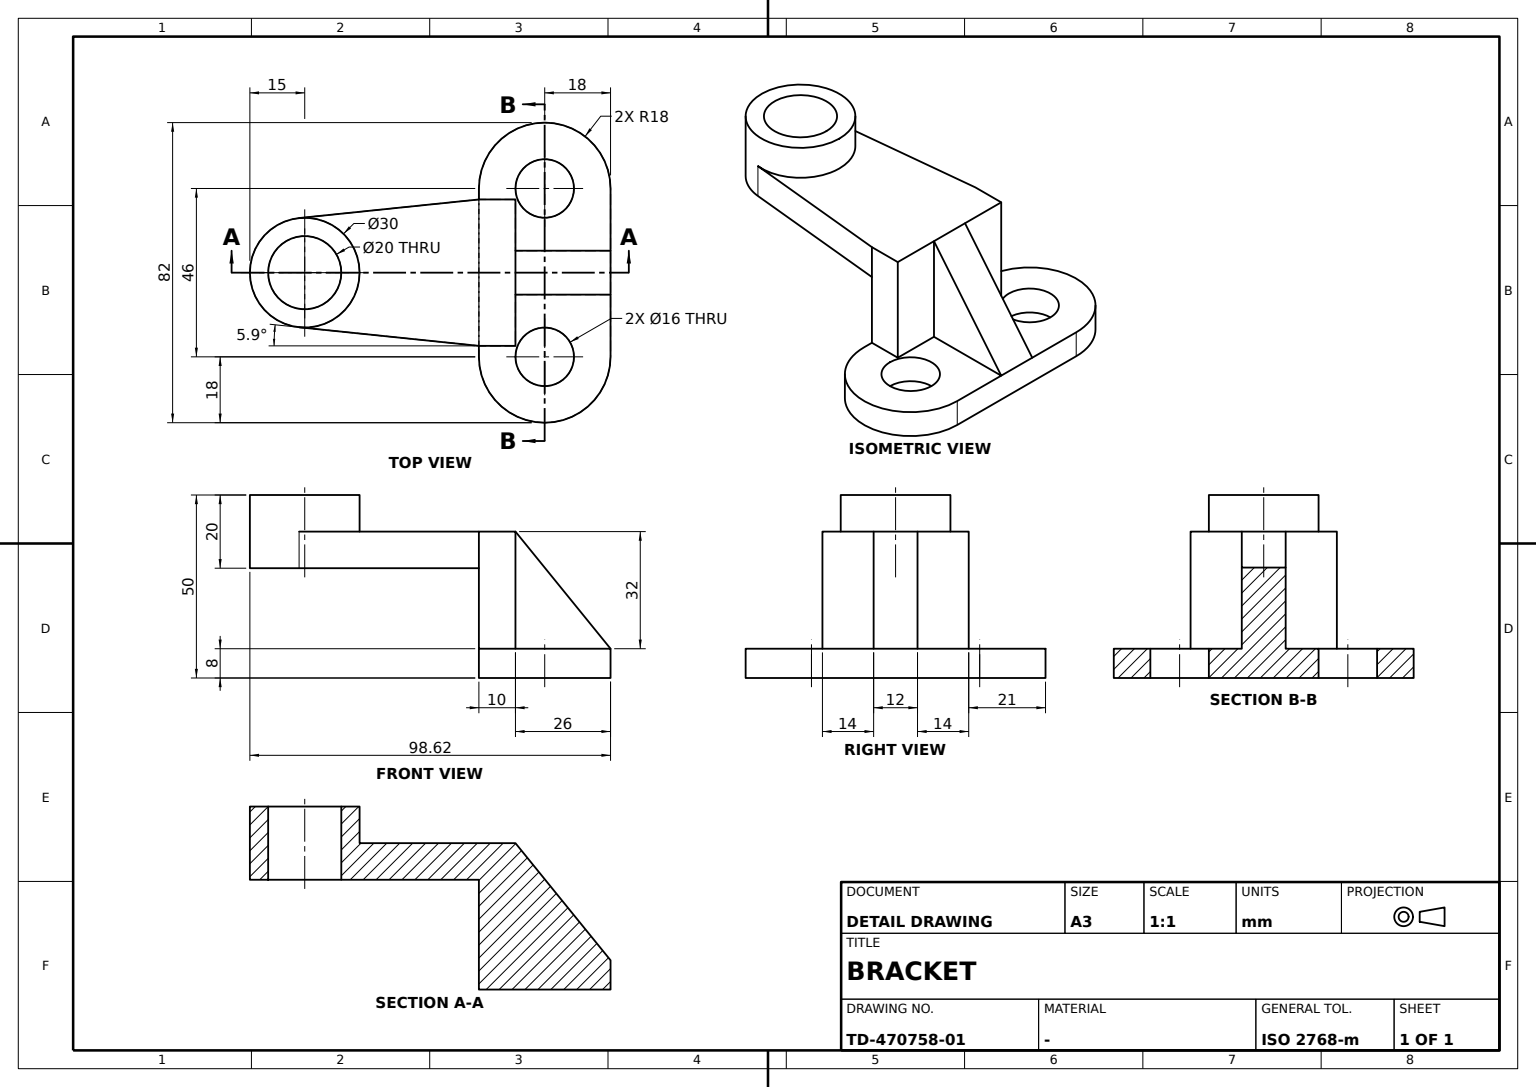
ISO-10303-21;
HEADER;
FILE_DESCRIPTION((''),'2;1');
FILE_NAME('','',(''),(''),'','','');
FILE_SCHEMA(('AUTOMOTIVE_DESIGN'));
ENDSEC;
DATA;
#1=APPLICATION_CONTEXT('');
#2=PRODUCT_CONTEXT('',#1,'mechanical');
#3=PRODUCT('','','',(#2));
#4=PRODUCT_DEFINITION_FORMATION('','',#3);
#5=PRODUCT_DEFINITION_CONTEXT('',#1,'design');
#6=PRODUCT_DEFINITION('','',#4,#5);
#7=PRODUCT_DEFINITION_SHAPE('','',#6);
#8=(LENGTH_UNIT()NAMED_UNIT(*)SI_UNIT(.MILLI.,.METRE.));
#9=(NAMED_UNIT(*)PLANE_ANGLE_UNIT()SI_UNIT($,.RADIAN.));
#10=(NAMED_UNIT(*)SI_UNIT($,.STERADIAN.)SOLID_ANGLE_UNIT());
#11=UNCERTAINTY_MEASURE_WITH_UNIT(LENGTH_MEASURE(0.005),#8,'distance_accuracy_value','');
#12=(GEOMETRIC_REPRESENTATION_CONTEXT(3)GLOBAL_UNCERTAINTY_ASSIGNED_CONTEXT((#11))GLOBAL_UNIT_ASSIGNED_CONTEXT((#8,#9,#10))REPRESENTATION_CONTEXT('',''));
#13=CARTESIAN_POINT('',(0.,-23.,0.));
#14=VERTEX_POINT('',#13);
#15=CARTESIAN_POINT('',(8.,-23.,0.));
#16=DIRECTION('',(0.,0.,-1.));
#17=DIRECTION('',(-1.,0.,0.));
#18=AXIS2_PLACEMENT_3D('',#15,#16,#17);
#19=CIRCLE('',#18,8.);
#20=EDGE_CURVE('',#14,#14,#19,.T.);
#21=ORIENTED_EDGE('',*,*,#20,.T.);
#22=EDGE_LOOP('',(#21));
#23=FACE_BOUND('',#22,.T.);
#24=CARTESIAN_POINT('',(0.,-6.,0.));
#25=VERTEX_POINT('',#24);
#26=CARTESIAN_POINT('',(26.,-6.,0.));
#27=VERTEX_POINT('',#26);
#28=DIRECTION('',(1.,0.,0.));
#29=VECTOR('',#28,1000.);
#30=LINE('',#24,#29);
#31=EDGE_CURVE('',#25,#27,#30,.T.);
#32=ORIENTED_EDGE('',*,*,#31,.F.);
#33=CARTESIAN_POINT('',(0.,-20.,0.));
#34=VERTEX_POINT('',#33);
#35=CARTESIAN_POINT('',(0.,0.,0.));
#36=DIRECTION('',(0.,1.,0.));
#37=VECTOR('',#36,1000.);
#38=LINE('',#35,#37);
#39=EDGE_CURVE('',#34,#25,#38,.T.);
#40=ORIENTED_EDGE('',*,*,#39,.F.);
#41=CARTESIAN_POINT('',(-10.,-20.,0.));
#42=VERTEX_POINT('',#41);
#43=VECTOR('',#17,1000.);
#44=LINE('',#33,#43);
#45=EDGE_CURVE('',#34,#42,#44,.T.);
#46=ORIENTED_EDGE('',*,*,#45,.T.);
#47=CARTESIAN_POINT('',(-10.,-23.,0.));
#48=VERTEX_POINT('',#47);
#49=CARTESIAN_POINT('',(-10.,0.,0.));
#50=DIRECTION('',(0.,-1.,0.));
#51=VECTOR('',#50,1000.);
#52=LINE('',#49,#51);
#53=EDGE_CURVE('',#42,#48,#52,.T.);
#54=ORIENTED_EDGE('',*,*,#53,.T.);
#55=CARTESIAN_POINT('',(26.,-23.,0.));
#56=VERTEX_POINT('',#55);
#57=CIRCLE('',#18,18.);
#58=EDGE_CURVE('',#56,#48,#57,.T.);
#59=ORIENTED_EDGE('',*,*,#58,.F.);
#60=CARTESIAN_POINT('',(26.,0.,0.));
#61=LINE('',#60,#37);
#62=EDGE_CURVE('',#56,#27,#61,.T.);
#63=ORIENTED_EDGE('',*,*,#62,.T.);
#64=EDGE_LOOP('',(#32,#40,#46,#54,#59,#63));
#65=FACE_BOUND('',#64,.T.);
#66=AXIS2_PLACEMENT_3D('',#35,#16,#17);
#67=PLANE('',#66);
#68=ADVANCED_FACE('',(#23,#65),#67,.F.);
#69=CARTESIAN_POINT('',(26.,-23.,-8.));
#70=VERTEX_POINT('',#69);
#71=CARTESIAN_POINT('',(26.,23.,-8.));
#72=VERTEX_POINT('',#71);
#73=CARTESIAN_POINT('',(26.,0.,-8.));
#74=LINE('',#73,#37);
#75=EDGE_CURVE('',#70,#72,#74,.T.);
#76=ORIENTED_EDGE('',*,*,#75,.F.);
#77=CARTESIAN_POINT('',(-10.,-23.,-8.));
#78=VERTEX_POINT('',#77);
#79=CARTESIAN_POINT('',(8.,-23.,-8.));
#80=AXIS2_PLACEMENT_3D('',#79,#16,#17);
#81=CIRCLE('',#80,18.);
#82=EDGE_CURVE('',#70,#78,#81,.T.);
#83=ORIENTED_EDGE('',*,*,#82,.T.);
#84=CARTESIAN_POINT('',(-10.,23.,-8.));
#85=VERTEX_POINT('',#84);
#86=CARTESIAN_POINT('',(-10.,0.,-8.));
#87=LINE('',#86,#51);
#88=EDGE_CURVE('',#85,#78,#87,.T.);
#89=ORIENTED_EDGE('',*,*,#88,.F.);
#90=CARTESIAN_POINT('',(8.,23.,-8.));
#91=AXIS2_PLACEMENT_3D('',#90,#16,#17);
#92=CIRCLE('',#91,18.);
#93=EDGE_CURVE('',#85,#72,#92,.T.);
#94=ORIENTED_EDGE('',*,*,#93,.T.);
#95=EDGE_LOOP('',(#76,#83,#89,#94));
#96=FACE_BOUND('',#95,.T.);
#97=CARTESIAN_POINT('',(0.,23.,-8.));
#98=VERTEX_POINT('',#97);
#99=CIRCLE('',#91,8.);
#100=EDGE_CURVE('',#98,#98,#99,.T.);
#101=ORIENTED_EDGE('',*,*,#100,.F.);
#102=EDGE_LOOP('',(#101));
#103=FACE_BOUND('',#102,.T.);
#104=CARTESIAN_POINT('',(0.,-23.,-8.));
#105=VERTEX_POINT('',#104);
#106=CIRCLE('',#80,8.);
#107=EDGE_CURVE('',#105,#105,#106,.T.);
#108=ORIENTED_EDGE('',*,*,#107,.F.);
#109=EDGE_LOOP('',(#108));
#110=FACE_BOUND('',#109,.T.);
#111=CARTESIAN_POINT('',(0.,0.,-8.));
#112=AXIS2_PLACEMENT_3D('',#111,#16,#28);
#113=PLANE('',#112);
#114=ADVANCED_FACE('',(#96,#103,#110),#113,.T.);
#115=CARTESIAN_POINT('',(-10.,-20.,32.));
#116=VERTEX_POINT('',#115);
#117=CARTESIAN_POINT('',(-10.,-20.,22.));
#118=VERTEX_POINT('',#117);
#119=VECTOR('',#16,1000.);
#120=LINE('',#41,#119);
#121=EDGE_CURVE('',#116,#118,#120,.T.);
#122=ORIENTED_EDGE('',*,*,#121,.F.);
#123=CARTESIAN_POINT('',(-59.162262,-14.920573,32.));
#124=VERTEX_POINT('',#123);
#125=DIRECTION('',(0.994704883,-0.102772541,0.));
#126=VECTOR('',#125,1000.);
#127=LINE('',#123,#126);
#128=EDGE_CURVE('',#124,#116,#127,.T.);
#129=ORIENTED_EDGE('',*,*,#128,.F.);
#130=CARTESIAN_POINT('',(-59.162262,-14.920573,22.));
#131=VERTEX_POINT('',#130);
#132=CARTESIAN_POINT('',(-59.162262,-14.920573,27.));
#133=DIRECTION('',(0.,0.,1.));
#134=VECTOR('',#133,1000.);
#135=LINE('',#132,#134);
#136=EDGE_CURVE('',#124,#131,#135,.F.);
#137=ORIENTED_EDGE('',*,*,#136,.T.);
#138=LINE('',#130,#126);
#139=EDGE_CURVE('',#131,#118,#138,.T.);
#140=ORIENTED_EDGE('',*,*,#139,.T.);
#141=EDGE_LOOP('',(#122,#129,#137,#140));
#142=FACE_BOUND('',#141,.T.);
#143=DIRECTION('',(0.102772541,0.994704883,0.));
#144=AXIS2_PLACEMENT_3D('',#123,#143,#125);
#145=PLANE('',#144);
#146=ADVANCED_FACE('',(#142),#145,.F.);
#147=CARTESIAN_POINT('',(-47.620674,0.,42.));
#148=VERTEX_POINT('',#147);
#149=CARTESIAN_POINT('',(-57.620674,0.,42.));
#150=AXIS2_PLACEMENT_3D('',#149,#133,#28);
#151=CIRCLE('',#150,10.);
#152=EDGE_CURVE('',#148,#148,#151,.T.);
#153=ORIENTED_EDGE('',*,*,#152,.T.);
#154=EDGE_LOOP('',(#153));
#155=FACE_BOUND('',#154,.T.);
#156=CARTESIAN_POINT('',(-47.620674,0.,22.));
#157=VERTEX_POINT('',#156);
#158=CARTESIAN_POINT('',(-57.620674,0.,22.));
#159=AXIS2_PLACEMENT_3D('',#158,#133,#28);
#160=CIRCLE('',#159,10.);
#161=EDGE_CURVE('',#157,#157,#160,.T.);
#162=ORIENTED_EDGE('',*,*,#161,.F.);
#163=EDGE_LOOP('',(#162));
#164=FACE_BOUND('',#163,.T.);
#165=CARTESIAN_POINT('',(-57.620674,0.,27.));
#166=AXIS2_PLACEMENT_3D('',#165,#133,#28);
#167=CYLINDRICAL_SURFACE('',#166,10.);
#168=ADVANCED_FACE('',(#155,#164),#167,.F.);
#169=CARTESIAN_POINT('',(-10.,-23.,-4.));
#170=LINE('',#169,#119);
#171=EDGE_CURVE('',#48,#78,#170,.T.);
#172=ORIENTED_EDGE('',*,*,#171,.T.);
#173=ORIENTED_EDGE('',*,*,#82,.F.);
#174=CARTESIAN_POINT('',(26.,-23.,-4.));
#175=LINE('',#174,#119);
#176=EDGE_CURVE('',#56,#70,#175,.T.);
#177=ORIENTED_EDGE('',*,*,#176,.F.);
#178=ORIENTED_EDGE('',*,*,#58,.T.);
#179=EDGE_LOOP('',(#172,#173,#177,#178));
#180=FACE_BOUND('',#179,.T.);
#181=CARTESIAN_POINT('',(8.,-23.,-4.));
#182=AXIS2_PLACEMENT_3D('',#181,#16,#28);
#183=CYLINDRICAL_SURFACE('',#182,18.);
#184=ADVANCED_FACE('',(#180),#183,.T.);
#185=CARTESIAN_POINT('',(0.,20.,0.));
#186=VERTEX_POINT('',#185);
#187=CARTESIAN_POINT('',(-10.,20.,0.));
#188=VERTEX_POINT('',#187);
#189=LINE('',#185,#43);
#190=EDGE_CURVE('',#186,#188,#189,.T.);
#191=ORIENTED_EDGE('',*,*,#190,.F.);
#192=CARTESIAN_POINT('',(0.,6.,0.));
#193=VERTEX_POINT('',#192);
#194=EDGE_CURVE('',#193,#186,#38,.T.);
#195=ORIENTED_EDGE('',*,*,#194,.F.);
#196=CARTESIAN_POINT('',(26.,6.,0.));
#197=VERTEX_POINT('',#196);
#198=LINE('',#192,#29);
#199=EDGE_CURVE('',#193,#197,#198,.T.);
#200=ORIENTED_EDGE('',*,*,#199,.T.);
#201=CARTESIAN_POINT('',(26.,23.,0.));
#202=VERTEX_POINT('',#201);
#203=EDGE_CURVE('',#197,#202,#61,.T.);
#204=ORIENTED_EDGE('',*,*,#203,.T.);
#205=CARTESIAN_POINT('',(-10.,23.,0.));
#206=VERTEX_POINT('',#205);
#207=CARTESIAN_POINT('',(8.,23.,0.));
#208=AXIS2_PLACEMENT_3D('',#207,#16,#17);
#209=CIRCLE('',#208,18.);
#210=EDGE_CURVE('',#206,#202,#209,.T.);
#211=ORIENTED_EDGE('',*,*,#210,.F.);
#212=EDGE_CURVE('',#206,#188,#52,.T.);
#213=ORIENTED_EDGE('',*,*,#212,.T.);
#214=EDGE_LOOP('',(#191,#195,#200,#204,#211,#213));
#215=FACE_BOUND('',#214,.T.);
#216=CARTESIAN_POINT('',(0.,23.,0.));
#217=VERTEX_POINT('',#216);
#218=CIRCLE('',#208,8.);
#219=EDGE_CURVE('',#217,#217,#218,.T.);
#220=ORIENTED_EDGE('',*,*,#219,.T.);
#221=EDGE_LOOP('',(#220));
#222=FACE_BOUND('',#221,.T.);
#223=ADVANCED_FACE('',(#215,#222),#67,.F.);
#224=CARTESIAN_POINT('',(0.,-6.,32.));
#225=VERTEX_POINT('',#224);
#226=CARTESIAN_POINT('',(0.,6.,32.));
#227=VERTEX_POINT('',#226);
#228=CARTESIAN_POINT('',(0.,0.,32.));
#229=LINE('',#228,#37);
#230=EDGE_CURVE('',#225,#227,#229,.T.);
#231=ORIENTED_EDGE('',*,*,#230,.F.);
#232=CARTESIAN_POINT('',(15.661176,-6.,12.724706));
#233=DIRECTION('',(-0.630592625,0.,0.776114));
#234=VECTOR('',#233,1000.);
#235=LINE('',#232,#234);
#236=EDGE_CURVE('',#27,#225,#235,.T.);
#237=ORIENTED_EDGE('',*,*,#236,.F.);
#238=EDGE_CURVE('',#27,#197,#61,.T.);
#239=ORIENTED_EDGE('',*,*,#238,.T.);
#240=CARTESIAN_POINT('',(15.661176,6.,12.724706));
#241=LINE('',#240,#234);
#242=EDGE_CURVE('',#197,#227,#241,.T.);
#243=ORIENTED_EDGE('',*,*,#242,.T.);
#244=EDGE_LOOP('',(#231,#237,#239,#243));
#245=FACE_BOUND('',#244,.T.);
#246=DIRECTION('',(-0.776114,0.,-0.630592625));
#247=AXIS2_PLACEMENT_3D('',#60,#246,#233);
#248=PLANE('',#247);
#249=ADVANCED_FACE('',(#245),#248,.F.);
#250=ORIENTED_EDGE('',*,*,#100,.T.);
#251=EDGE_LOOP('',(#250));
#252=FACE_BOUND('',#251,.T.);
#253=ORIENTED_EDGE('',*,*,#219,.F.);
#254=EDGE_LOOP('',(#253));
#255=FACE_BOUND('',#254,.T.);
#256=CARTESIAN_POINT('',(8.,23.,-4.));
#257=AXIS2_PLACEMENT_3D('',#256,#16,#28);
#258=CYLINDRICAL_SURFACE('',#257,8.);
#259=ADVANCED_FACE('',(#252,#255),#258,.F.);
#260=ORIENTED_EDGE('',*,*,#53,.F.);
#261=LINE('',#41,#134);
#262=EDGE_CURVE('',#42,#118,#261,.T.);
#263=ORIENTED_EDGE('',*,*,#262,.T.);
#264=CARTESIAN_POINT('',(-10.,20.,22.));
#265=VERTEX_POINT('',#264);
#266=CARTESIAN_POINT('',(-10.,0.,22.));
#267=LINE('',#266,#51);
#268=EDGE_CURVE('',#265,#118,#267,.T.);
#269=ORIENTED_EDGE('',*,*,#268,.F.);
#270=LINE('',#187,#134);
#271=EDGE_CURVE('',#188,#265,#270,.T.);
#272=ORIENTED_EDGE('',*,*,#271,.F.);
#273=ORIENTED_EDGE('',*,*,#212,.F.);
#274=CARTESIAN_POINT('',(-10.,23.,-4.));
#275=LINE('',#274,#119);
#276=EDGE_CURVE('',#206,#85,#275,.T.);
#277=ORIENTED_EDGE('',*,*,#276,.T.);
#278=ORIENTED_EDGE('',*,*,#88,.T.);
#279=ORIENTED_EDGE('',*,*,#171,.F.);
#280=EDGE_LOOP('',(#260,#263,#269,#272,#273,#277,#278,#279));
#281=FACE_BOUND('',#280,.T.);
#282=AXIS2_PLACEMENT_3D('',#49,#17,#133);
#283=PLANE('',#282);
#284=ADVANCED_FACE('',(#281),#283,.T.);
#285=ORIENTED_EDGE('',*,*,#238,.F.);
#286=ORIENTED_EDGE('',*,*,#62,.F.);
#287=ORIENTED_EDGE('',*,*,#176,.T.);
#288=ORIENTED_EDGE('',*,*,#75,.T.);
#289=CARTESIAN_POINT('',(26.,23.,-4.));
#290=LINE('',#289,#119);
#291=EDGE_CURVE('',#202,#72,#290,.T.);
#292=ORIENTED_EDGE('',*,*,#291,.F.);
#293=ORIENTED_EDGE('',*,*,#203,.F.);
#294=EDGE_LOOP('',(#285,#286,#287,#288,#292,#293));
#295=FACE_BOUND('',#294,.T.);
#296=AXIS2_PLACEMENT_3D('',#55,#17,#36);
#297=PLANE('',#296);
#298=ADVANCED_FACE('',(#295),#297,.F.);
#299=ORIENTED_EDGE('',*,*,#199,.F.);
#300=LINE('',#192,#119);
#301=EDGE_CURVE('',#227,#193,#300,.T.);
#302=ORIENTED_EDGE('',*,*,#301,.F.);
#303=ORIENTED_EDGE('',*,*,#242,.F.);
#304=EDGE_LOOP('',(#299,#302,#303));
#305=FACE_BOUND('',#304,.T.);
#306=AXIS2_PLACEMENT_3D('',#192,#36,#17);
#307=PLANE('',#306);
#308=ADVANCED_FACE('',(#305),#307,.T.);
#309=ORIENTED_EDGE('',*,*,#301,.T.);
#310=ORIENTED_EDGE('',*,*,#194,.T.);
#311=CARTESIAN_POINT('',(0.,20.,32.));
#312=VERTEX_POINT('',#311);
#313=LINE('',#185,#119);
#314=EDGE_CURVE('',#312,#186,#313,.T.);
#315=ORIENTED_EDGE('',*,*,#314,.F.);
#316=EDGE_CURVE('',#227,#312,#229,.T.);
#317=ORIENTED_EDGE('',*,*,#316,.F.);
#318=EDGE_LOOP('',(#309,#310,#315,#317));
#319=FACE_BOUND('',#318,.T.);
#320=AXIS2_PLACEMENT_3D('',#228,#28,#16);
#321=PLANE('',#320);
#322=ADVANCED_FACE('',(#319),#321,.T.);
#323=CARTESIAN_POINT('',(-10.,20.,32.));
#324=VERTEX_POINT('',#323);
#325=LINE('',#311,#29);
#326=EDGE_CURVE('',#324,#312,#325,.T.);
#327=ORIENTED_EDGE('',*,*,#326,.F.);
#328=CARTESIAN_POINT('',(-59.162262,14.920573,32.));
#329=VERTEX_POINT('',#328);
#330=DIRECTION('',(0.994704883,0.102772541,0.));
#331=VECTOR('',#330,1000.);
#332=LINE('',#328,#331);
#333=EDGE_CURVE('',#329,#324,#332,.T.);
#334=ORIENTED_EDGE('',*,*,#333,.F.);
#335=CARTESIAN_POINT('',(-57.620674,0.,32.));
#336=AXIS2_PLACEMENT_3D('',#335,#133,#28);
#337=CIRCLE('',#336,15.);
#338=EDGE_CURVE('',#124,#329,#337,.T.);
#339=ORIENTED_EDGE('',*,*,#338,.F.);
#340=ORIENTED_EDGE('',*,*,#128,.T.);
#341=CARTESIAN_POINT('',(0.,-20.,32.));
#342=VERTEX_POINT('',#341);
#343=LINE('',#341,#29);
#344=EDGE_CURVE('',#116,#342,#343,.T.);
#345=ORIENTED_EDGE('',*,*,#344,.T.);
#346=EDGE_CURVE('',#342,#225,#229,.T.);
#347=ORIENTED_EDGE('',*,*,#346,.T.);
#348=ORIENTED_EDGE('',*,*,#230,.T.);
#349=ORIENTED_EDGE('',*,*,#316,.T.);
#350=EDGE_LOOP('',(#327,#334,#339,#340,#345,#347,#348,#349));
#351=FACE_BOUND('',#350,.T.);
#352=CARTESIAN_POINT('',(-10.,0.,32.));
#353=AXIS2_PLACEMENT_3D('',#352,#133,#28);
#354=PLANE('',#353);
#355=ADVANCED_FACE('',(#351),#354,.T.);
#356=CARTESIAN_POINT('',(-42.620674,0.,42.));
#357=VERTEX_POINT('',#356);
#358=CIRCLE('',#150,15.);
#359=EDGE_CURVE('',#357,#357,#358,.T.);
#360=ORIENTED_EDGE('',*,*,#359,.F.);
#361=EDGE_LOOP('',(#360));
#362=FACE_BOUND('',#361,.T.);
#363=CARTESIAN_POINT('',(-59.162262,14.920573,22.));
#364=VERTEX_POINT('',#363);
#365=CIRCLE('',#159,15.);
#366=EDGE_CURVE('',#364,#131,#365,.T.);
#367=ORIENTED_EDGE('',*,*,#366,.T.);
#368=ORIENTED_EDGE('',*,*,#136,.F.);
#369=ORIENTED_EDGE('',*,*,#338,.T.);
#370=CARTESIAN_POINT('',(-59.162262,14.920573,27.));
#371=LINE('',#370,#134);
#372=EDGE_CURVE('',#329,#364,#371,.F.);
#373=ORIENTED_EDGE('',*,*,#372,.T.);
#374=EDGE_LOOP('',(#367,#368,#369,#373));
#375=FACE_BOUND('',#374,.T.);
#376=CYLINDRICAL_SURFACE('',#166,15.);
#377=ADVANCED_FACE('',(#362,#375),#376,.T.);
#378=ORIENTED_EDGE('',*,*,#20,.F.);
#379=EDGE_LOOP('',(#378));
#380=FACE_BOUND('',#379,.T.);
#381=ORIENTED_EDGE('',*,*,#107,.T.);
#382=EDGE_LOOP('',(#381));
#383=FACE_BOUND('',#382,.T.);
#384=CYLINDRICAL_SURFACE('',#182,8.);
#385=ADVANCED_FACE('',(#380,#383),#384,.F.);
#386=ORIENTED_EDGE('',*,*,#346,.F.);
#387=LINE('',#33,#119);
#388=EDGE_CURVE('',#342,#34,#387,.T.);
#389=ORIENTED_EDGE('',*,*,#388,.T.);
#390=ORIENTED_EDGE('',*,*,#39,.T.);
#391=LINE('',#24,#119);
#392=EDGE_CURVE('',#225,#25,#391,.T.);
#393=ORIENTED_EDGE('',*,*,#392,.F.);
#394=EDGE_LOOP('',(#386,#389,#390,#393));
#395=FACE_BOUND('',#394,.T.);
#396=ADVANCED_FACE('',(#395),#321,.T.);
#397=ORIENTED_EDGE('',*,*,#31,.T.);
#398=ORIENTED_EDGE('',*,*,#236,.T.);
#399=ORIENTED_EDGE('',*,*,#392,.T.);
#400=EDGE_LOOP('',(#397,#398,#399));
#401=FACE_BOUND('',#400,.T.);
#402=AXIS2_PLACEMENT_3D('',#24,#36,#17);
#403=PLANE('',#402);
#404=ADVANCED_FACE('',(#401),#403,.F.);
#405=ORIENTED_EDGE('',*,*,#139,.F.);
#406=ORIENTED_EDGE('',*,*,#366,.F.);
#407=LINE('',#363,#331);
#408=EDGE_CURVE('',#364,#265,#407,.T.);
#409=ORIENTED_EDGE('',*,*,#408,.T.);
#410=ORIENTED_EDGE('',*,*,#268,.T.);
#411=EDGE_LOOP('',(#405,#406,#409,#410));
#412=FACE_BOUND('',#411,.T.);
#413=ORIENTED_EDGE('',*,*,#161,.T.);
#414=EDGE_LOOP('',(#413));
#415=FACE_BOUND('',#414,.T.);
#416=CARTESIAN_POINT('',(0.,0.,22.));
#417=AXIS2_PLACEMENT_3D('',#416,#133,#28);
#418=PLANE('',#417);
#419=ADVANCED_FACE('',(#412,#415),#418,.F.);
#420=ORIENTED_EDGE('',*,*,#276,.F.);
#421=ORIENTED_EDGE('',*,*,#210,.T.);
#422=ORIENTED_EDGE('',*,*,#291,.T.);
#423=ORIENTED_EDGE('',*,*,#93,.F.);
#424=EDGE_LOOP('',(#420,#421,#422,#423));
#425=FACE_BOUND('',#424,.T.);
#426=CYLINDRICAL_SURFACE('',#257,18.);
#427=ADVANCED_FACE('',(#425),#426,.T.);
#428=ORIENTED_EDGE('',*,*,#408,.F.);
#429=ORIENTED_EDGE('',*,*,#372,.F.);
#430=ORIENTED_EDGE('',*,*,#333,.T.);
#431=LINE('',#323,#119);
#432=EDGE_CURVE('',#324,#265,#431,.T.);
#433=ORIENTED_EDGE('',*,*,#432,.T.);
#434=EDGE_LOOP('',(#428,#429,#430,#433));
#435=FACE_BOUND('',#434,.T.);
#436=DIRECTION('',(-0.102772541,0.994704883,0.));
#437=AXIS2_PLACEMENT_3D('',#328,#436,#330);
#438=PLANE('',#437);
#439=ADVANCED_FACE('',(#435),#438,.T.);
#440=ORIENTED_EDGE('',*,*,#359,.T.);
#441=EDGE_LOOP('',(#440));
#442=FACE_BOUND('',#441,.T.);
#443=ORIENTED_EDGE('',*,*,#152,.F.);
#444=EDGE_LOOP('',(#443));
#445=FACE_BOUND('',#444,.T.);
#446=CARTESIAN_POINT('',(0.,0.,42.));
#447=AXIS2_PLACEMENT_3D('',#446,#133,#28);
#448=PLANE('',#447);
#449=ADVANCED_FACE('',(#442,#445),#448,.T.);
#450=ORIENTED_EDGE('',*,*,#121,.T.);
#451=ORIENTED_EDGE('',*,*,#262,.F.);
#452=ORIENTED_EDGE('',*,*,#45,.F.);
#453=ORIENTED_EDGE('',*,*,#388,.F.);
#454=ORIENTED_EDGE('',*,*,#344,.F.);
#455=EDGE_LOOP('',(#450,#451,#452,#453,#454));
#456=FACE_BOUND('',#455,.T.);
#457=AXIS2_PLACEMENT_3D('',#33,#36,#17);
#458=PLANE('',#457);
#459=ADVANCED_FACE('',(#456),#458,.F.);
#460=ORIENTED_EDGE('',*,*,#271,.T.);
#461=ORIENTED_EDGE('',*,*,#432,.F.);
#462=ORIENTED_EDGE('',*,*,#326,.T.);
#463=ORIENTED_EDGE('',*,*,#314,.T.);
#464=ORIENTED_EDGE('',*,*,#190,.T.);
#465=EDGE_LOOP('',(#460,#461,#462,#463,#464));
#466=FACE_BOUND('',#465,.T.);
#467=AXIS2_PLACEMENT_3D('',#185,#36,#17);
#468=PLANE('',#467);
#469=ADVANCED_FACE('',(#466),#468,.T.);
#470=CLOSED_SHELL('',(#68,#114,#146,#168,#184,#223,#249,#259,#284,#298,#308,#322,#355,#377,#385,#396,#404,#419,#427,#439,#449,#459,#469));
#471=MANIFOLD_SOLID_BREP('',#470);
#472=ADVANCED_BREP_SHAPE_REPRESENTATION('',(#471),#12);
#473=SHAPE_DEFINITION_REPRESENTATION(#7,#472);
ENDSEC;
END-ISO-10303-21;
